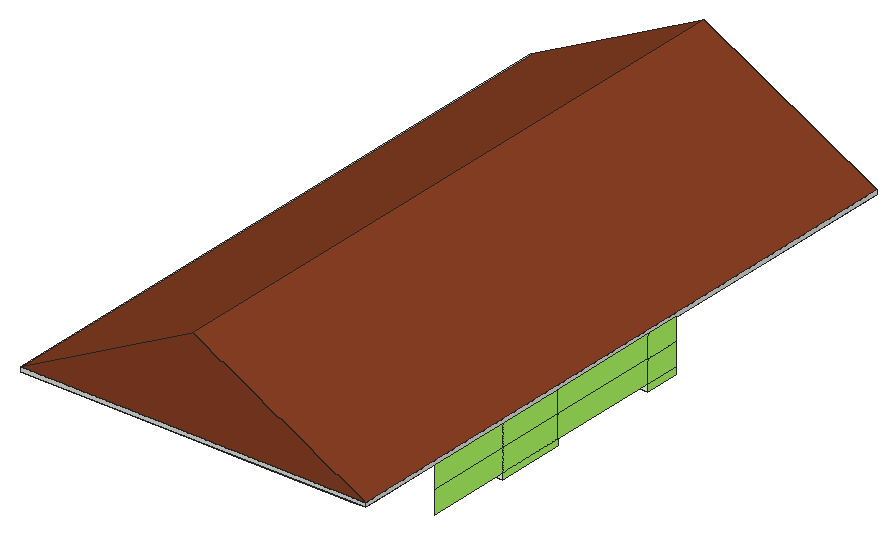
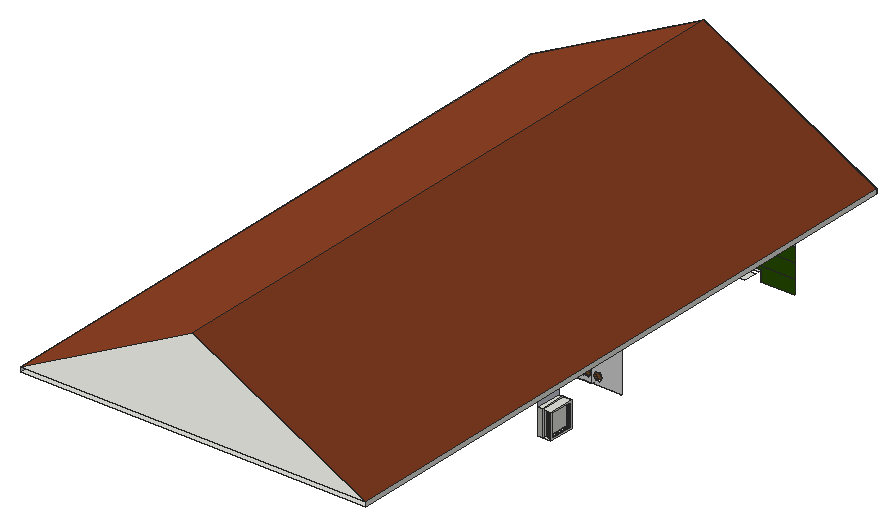
# SketchUp Ruby script. Lengths in inches.
U = 1.inch
M = Sketchup.active_model
def pt(a) = Geom::Point3d.new(a.map { |v| v * U })
def face(e, loops, mat)
  f = e.add_face(loops[0].map { |a| pt(a) })
  loops[1..].each { |l| e.add_face(l.map { |a| pt(a) }).erase! }
  f.material = f.back_material = mat if mat
  f
end
# faces: each face lists its corners as indices into pts; further lists are holes
def faces(e, pts, list, mat = nil) = list.each { |f| face(e, (f[0].is_a?(Array) ? f : [f]).map { |l| l.map { |i| pts[i] } }, mat) }
# xy, xz, yz: faces in a plane at the given z, y or x. An outline is a flat list of corners, or four numbers for a rectangle; further outlines are holes
def ring(l) = l.size == 4 ? [[l[0], l[1]], [l[2], l[1]], [l[2], l[3]], [l[0], l[3]]] : l.each_slice(2).to_a
def flat(e, list, mat, &to3) = list.each { |f| face(e, (f[0].is_a?(Array) ? f : [f]).map { |l| ring(l).map { |u, v| to3.(u, v) } }, mat) }
def xy(e, z, list, mat = nil) = flat(e, list, mat) { |x, y| [x, y, z] }
def xz(e, y, list, mat = nil) = flat(e, list, mat) { |x, z| [x, y, z] }
def yz(e, x, list, mat = nil) = flat(e, list, mat) { |y, z| [x, y, z] }
def lines(e, pts, list) = list.each { |a, b| e.add_line(pt(pts[a]), pt(pts[b])) }
# prism: a flat outline (further loops are holes) pulled along v
def prism(e, loops, v, mat = nil)
  f = face(e, loops, mat); d = Geom::Vector3d.new(v.map { |x| x * U })
  f.pushpull(f.normal.samedirection?(d) ? d.length : -d.length)
end
def box(e, o, s, mat = nil) = prism(e, [[o, [o[0] + s[0], o[1], o[2]], [o[0] + s[0], o[1] + s[1], o[2]], [o[0], o[1] + s[1], o[2]]]], [0, 0, s[2]], mat)
def at(x, y, z, deg = 0) = Geom::Transformation.translation(pt([x, y, z])) * Geom::Transformation.rotation(ORIGIN, Z_AXIS, deg.degrees)
def axes(o, x, y, z) = Geom::Transformation.new([*x, 0, *y, 0, *z, 0, *pt(o).to_a, 1])
def part(name) = M.definitions.add(name)
# library, detail: a bought-in or finely detailed component or shape, given as its bounding box
def library(name, o, s) = part(name).tap { |d| box(d.entities, o, s) }
def detail(e, o, s) = box(e.add_group.entities, o, s)
def put(e, d, t, mat = nil) = e.add_instance(d, t).tap { |i| i.material = mat if mat }
def group(e, t, mat = nil) = e.add_group.tap { |g| g.transformation = t; g.material = mat if mat }.entities
root = M.entities
M.materials.add("[Color F01]").color = [47, 96, 0]
M.materials.add("[Color F03]").color = [178, 255, 101]
M.materials.add("[Color K01]").color = [255, 204, 255]
M.materials.add("[Color M00]").color = [255, 255, 255]
M.materials.add("[Color M09]").color = [0, 0, 0]
M.materials.add("[Marble Carrara Floor Tile]").color = [204, 208, 219]
M.materials.add("[Roofing Tile Spanish]").color = [138, 64, 36]
M.materials.add("[Wood Cherry Original]").color = [152, 86, 42]
M.materials.add("[Wood Floor Parquet]").color = [145, 89, 39]
c1 = part("Copyright 2018, ")
xy(c1.entities,0.05,[[[19.06,0,19.06,9.82,21.3125,9.82,22.13,9.76,22.85,9.6,23.48,9.33,24,8.95,24.43,8.48,24.73,7.92,24.91,7.28,24.97,6.54,24.91,5.85,24.74,5.21,24.46,4.64,24.0625,4.14,23.58,3.73,23.03,3.4375,22.42,3.26,21.75,3.2,21.1,3.27,20.375,3.48,20.375,0],[21.62,4.3125,22.05,4.35,22.4375,4.47,22.79,4.66,23.09,4.94,23.34,5.28,23.52,5.66,23.63,6.09,23.67,6.56,23.6,7.16,23.4,7.68,23.08,8.1,22.66,8.39,22.08,8.56,21.28,8.61,20.375,8.61,20.375,4.61,20.98,4.39]],[25.77,0,27.98,4.71,25.47,9.82,26.9375,9.82,28.69,6.14,30.375,9.82,31.82,9.82,27.21,0],[[43.77,0,43.11,0.03,42.52,0.14,41.99,0.3125,41.54,0.55,41.18,0.86,40.92,1.2,40.77,1.6,40.71,2.04,40.82,2.64,41.12,3.13,41.63,3.5,42.35,3.75,41.86,4.16,41.74,4.37,41.7,4.57,41.77,4.87,41.98,5.14,42.3,5.36,42.73,5.51,42.1,5.88,41.65,6.34,41.38,6.91,41.29,7.57,41.34,8.0625,41.48,8.5,41.72,8.88,42.05,9.21,42.47,9.48,42.95,9.67,43.5,9.78,44.13,9.82,46.81,9.82,46.81,8.8125,45.49,8.8125,46.02,8.11,46.13,7.77,46.17,7.38,46.1,6.875,45.88,6.38,45.55,5.94,45.13,5.625,44.53,5.39,43.64,5.21,43.09,5.03,42.96,4.89,42.91,4.71,42.98,4.5,43.18,4.34,44.17,4.04,45.71,3.625,46.33,3.2,46.67,2.67,46.79,2.03,46.74,1.59,46.59,1.2,46.33,0.85,45.97,0.55,45.52,0.31,45.01,0.14,44.42,0.03],[43.74,1.02,44.5,1.09,45.0625,1.28,45.42,1.58,45.53,1.99,45.5,2.2,45.39,2.4,44.94,2.72,44.26,2.9375,43.41,3.01,42.82,2.94,42.34,2.73,42.03,2.42,41.93,2.03,42.04,1.59,42.38,1.28,42.95,1.09],[43.72,6.34,44.22,6.42,44.63,6.67,44.91,7.05,45,7.51,44.9,7.98,44.63,8.36,44.22,8.61,43.71,8.7,43.23,8.61,42.82,8.35,42.54,7.96,42.45,7.5,42.54,7.04,42.8125,6.67,43.22,6.42]],[180.16,0,182.36,4.71,179.85,9.82,181.32,9.82,183.07,6.14,184.75,9.82,186.2,9.82,181.59,0],[[219.8,0,219.13,0.03,218.54,0.14,218.02,0.3125,217.57,0.55,217.21,0.86,216.95,1.2,216.79,1.6,216.74,2.04,216.84,2.64,217.15,3.13,217.66,3.5,218.375,3.75,217.89,4.16,217.77,4.37,217.72,4.57,217.79,4.87,218,5.14,218.33,5.36,218.76,5.51,218.13,5.88,217.68,6.34,217.41,6.91,217.32,7.57,217.37,8.0625,217.51,8.5,217.75,8.88,218.08,9.21,218.5,9.48,218.98,9.67,219.53,9.78,220.16,9.82,222.83,9.82,222.83,8.8125,221.52,8.8125,222.05,8.11,222.16,7.77,222.2,7.38,222.125,6.875,221.91,6.38,221.58,5.94,221.16,5.625,220.5625,5.39,219.67,5.21,219.12,5.03,218.99,4.89,218.94,4.71,219.01,4.5,219.21,4.34,220.2,4.04,221.73,3.625,222.35,3.2,222.7,2.67,222.82,2.03,222.77,1.59,222.61,1.2,222.36,0.85,222,0.55,221.55,0.31,221.03,0.14,220.45,0.03],[219.77,1.02,220.53,1.09,221.09,1.28,221.44,1.58,221.5625,1.99,221.52,2.2,221.41,2.4,220.97,2.72,220.29,2.9375,219.43,3.01,218.84,2.94,218.37,2.73,218.0625,2.42,217.96,2.03,218.07,1.59,218.41,1.28,218.98,1.09],[219.75,6.34,220.25,6.42,220.66,6.67,220.93,7.05,221.02,7.51,220.93,7.98,220.66,8.36,220.24,8.61,219.74,8.7,219.25,8.61,218.85,8.35,218.57,7.96,218.48,7.5,218.57,7.04,218.84,6.67,219.25,6.42]],
  [92.62,1.6,92.62,1.87,92.89,2.17,93.07,2.48,93.22,3.3125,92.89,3.45,92.65,3.66,92.51,3.92,92.47,4.24,92.53,4.6,92.72,4.9,93.01,5.11,93.34,5.18,93.73,5.08,94.04,4.8,94.25,4.36,94.32,3.82,94.2,3.09,93.87,2.45,93.33,1.9375],[6.01,3.2,5.21,3.24,4.48,3.37,3.81,3.58,3.2,3.87,2.66,4.23,2.17,4.66,1.74,5.14,1.38,5.7,1.08,6.29,0.875,6.91,0.75,7.55,0.71,8.22,0.8,9.25,1.09,10.2,1.57,11.07,2.24,11.84,3.06,12.49,3.96,12.95,4.95,13.22,6.04,13.3125,6.83,13.26,7.68,13.11,8.5625,12.86,9.49,12.5,9.49,10.98,8.63,11.42,7.78,11.72,6.9375,11.91,6.11,11.97,5.29,11.9,4.55,11.7,3.89,11.37,3.29,10.9,2.8,10.33,2.45,9.7,2.24,8.99,2.17,8.22,2.24,7.44,2.45,6.74,2.79,6.11,3.27,5.55,3.86,5.09,4.53,4.76,5.27,4.57,6.09,4.5,6.98,4.57,7.87,4.78,8.74,5.12,9.6,5.6,9.6,4.05,8.79,3.68,7.92,3.41,6.99,3.25],[[14.21,3.2,13.51,3.26,12.87,3.4375,12.29,3.73,11.77,4.14,11.34,4.65,11.03,5.21,10.85,5.82,10.78,6.5,10.85,7.1875,11.03,7.81,11.34,8.375,11.78,8.88,12.31,9.3,12.9,9.59,13.55,9.77,14.27,9.83,14.98,9.77,15.63,9.59,16.21,9.29,16.73,8.87,17.16,8.36,17.47,7.79,17.66,7.16,17.72,6.47,17.66,5.79,17.47,5.18,17.16,4.625,16.72,4.13,16.19,3.72,15.6,3.43,14.9375,3.26],[14.25,4.4,14.71,4.44,15.12,4.55,15.48,4.74,15.81,5,16.07,5.32,16.26,5.68,16.37,6.08,16.41,6.53,16.37,6.97,16.25,7.375,16.06,7.74,15.78,8.0625,15.45,8.33,15.07,8.52,14.65,8.63,14.2,8.67,13.76,8.63,13.36,8.52,13,8.33,12.68,8.0625,12.42,7.74,12.23,7.37,12.12,6.97,12.08,6.52,12.12,6.07,12.24,5.67,12.43,5.31,12.69,4.99,13.02,4.73,13.39,4.55,13.8,4.44]],[57.3125,3.2,56.51,3.33,55.84,3.72,55.54,4.07,55.34,4.58,55.26,5.77,55.26,8.66,54.13,8.66,54.13,8.78,56.54,11.16,56.54,9.82,58.6,9.82,58.6,8.66,56.54,8.66,56.54,5.48,56.6,4.99,56.78,4.64,57.06,4.43,57.47,4.36,58.18,4.48,58.93,4.82,58.93,3.62,58.16,3.31],[[88.3125,3.2,87.67,3.25,87.08,3.41,86.54,3.66,86.06,4.02,85.66,4.45,85.37,4.93,85.2,5.46,85.14,6.04,85.23,6.75,85.49,7.37,85.93,7.91,86.54,8.36,86,8.86,85.64,9.37,85.4375,9.91,85.37,10.54,85.43,11.1,85.59,11.61,85.86,12.08,86.24,12.51,86.7,12.86,87.21,13.11,87.76,13.26,88.37,13.3125,88.96,13.26,89.51,13.11,90.01,12.86,90.46,12.51,90.83,12.09,91.09,11.62,91.25,11.1,91.31,10.54,91.23,9.91,91,9.33,90.62,8.82,90.08,8.36,90.68,7.91,91.11,7.38,91.36,6.75,91.45,6.02,91.39,5.4375,91.23,4.91,90.95,4.43,90.56,4,90.08,3.65,89.55,3.4,88.96,3.25],[88.33,4.54,89,4.64,89.54,4.94,89.9,5.39,90.02,5.96,90.02,6.11,89.9,6.72,89.54,7.21,88.98,7.53,88.28,7.64,87.6,7.53,87.05,7.21,86.69,6.71,86.57,6.09,86.69,5.47,87.06,4.98,87.62,4.65],[88.35,9.02,88.95,9.125,89.45,9.45,89.79,9.93,89.9,10.49,89.79,11.08,89.46,11.55,88.96,11.87,88.34,11.97,87.72,11.87,87.22,11.5625,86.89,11.09,86.78,10.51,86.89,9.9375,87.24,9.46,87.75,9.13]],
  [[113.29,3.2,112.92,3.24,112.64,3.36,112.43,3.57,112.32,3.85,111.9,3.57,111.47,3.375,111.03,3.26,110.57,3.22,109.95,3.33,109.44,3.66,109.1,4.17,108.99,4.79,109.1,5.375,109.43,5.89,109.97,6.32,110.6875,6.66,112.33,7.22,112.33,7.57,112.26,8.08,112.04,8.45,111.67,8.67,111.16,8.74,110.64,8.67,110.12,8.47,109.61,8.13,109.11,7.65,109.11,9.06,109.53,9.45,110.02,9.72,110.6,9.89,111.27,9.94,111.77,9.91,112.21,9.81,112.61,9.63,112.95,9.39,113.34,8.92,113.55,8.34,113.6,7.22,113.6,4.46,113.65,4.21,113.82,4.13,114.12,4.21,114.55,4.47,114.55,3.6875,113.85,3.3],[111.19,4.1,111.79,4.22,112.33,4.6,112.33,6.53,111.47,6.2,110.91,5.9375,110.54,5.67,110.34,5.375,110.27,5.01,110.33,4.64,110.53,4.35,110.82,4.16]],[121.02,3.2,120.43,3.28,119.88,3.51,119.43,3.87,119.1,4.34,118.9,5.04,118.83,6.09,118.83,9.82,120.12,9.82,120.12,6.11,120.19,5.24,120.41,4.68,120.82,4.38,121.44,4.28,121.88,4.33,122.29,4.5,122.66,4.78,123,5.17,123,9.82,124.29,9.82,124.29,3.3125,123,3.3125,123,4.15,122.5625,3.75,122.07,3.45,121.54,3.26],[[156.36,3.2,155.99,3.24,155.7,3.36,155.5,3.57,155.39,3.85,154.97,3.57,154.54,3.375,154.1,3.26,153.64,3.22,153.02,3.33,152.51,3.66,152.17,4.17,152.06,4.79,152.17,5.375,152.5,5.89,153.03,6.32,153.75,6.66,155.4,7.22,155.4,7.57,155.33,8.08,155.11,8.45,154.74,8.67,154.23,8.74,153.7,8.67,153.1875,8.47,152.68,8.13,152.18,7.65,152.18,9.06,152.59,9.45,153.09,9.72,153.67,9.89,154.33,9.94,154.83,9.91,155.28,9.81,155.68,9.63,156.02,9.39,156.4,8.92,156.62,8.34,156.66,7.22,156.66,4.46,156.72,4.21,156.89,4.13,157.1875,4.21,157.62,4.47,157.62,3.6875,156.92,3.3],[154.26,4.1,154.85,4.22,155.4,4.6,155.4,6.53,154.54,6.2,153.98,5.9375,153.61,5.67,153.4,5.375,153.34,5.01,153.4,4.64,153.59,4.35,153.89,4.16]],[161.74,3.2,161.01,3.26,160.37,3.43,159.8,3.71,159.3,4.11,158.91,4.6,158.62,5.16,158.45,5.81,158.4,6.53,158.45,7.26,158.62,7.92,158.89,8.5,159.28,9,159.76,9.41,160.3,9.71,160.92,9.88,161.6,9.94,162.51,9.85,163.49,9.49,163.49,8.12,162.55,8.59,161.68,8.74,161.27,8.7,160.89,8.59,160.55,8.4,160.25,8.13,160.01,7.8,159.84,7.4375,159.73,7.02,159.7,6.57,159.73,6.1,159.85,5.68,160.04,5.31,160.3,4.99,160.63,4.73,161.01,4.55,161.44,4.4375,161.93,4.4,162.73,4.51,163.63,4.83,163.63,3.5625,162.67,3.29],[[178.37,3.2,178,3.24,177.71,3.36,177.51,3.57,177.39,3.85,176.98,3.57,176.55,3.375,176.1,3.26,175.65,3.22,175.02,3.33,174.52,3.66,174.18,4.17,174.0625,4.79,174.17,5.375,174.51,5.89,175.04,6.32,175.76,6.66,177.41,7.22,177.41,7.57,177.33,8.08,177.11,8.45,176.75,8.67,176.23,8.74,175.71,8.67,175.19,8.47,174.6875,8.13,174.18,7.65,174.18,9.06,174.6,9.45,175.1,9.72,175.68,9.89,176.34,9.94,176.84,9.91,177.29,9.81,177.68,9.63,178.03,9.39,178.41,8.92,178.625,8.34,178.67,7.22,178.67,4.46,178.73,4.21,178.9,4.13,179.2,4.21,179.625,4.47,179.625,3.6875,178.92,3.3],[176.27,4.1,176.86,4.22,177.41,4.6,177.41,6.53,176.54,6.2,175.98,5.9375,175.61,5.67,175.41,5.375,175.34,5.01,175.41,4.64,175.6,4.35,175.9,4.16]],
  [210.76,3.2,209.73,3.33,208.59,3.78,208.59,5.17,209.71,4.55,210.23,4.37,210.66,4.3125,211.04,4.36,211.36,4.51,211.57,4.73,211.65,4.98,211.6,5.24,211.46,5.45,210.65,5.99,209.62,6.64,209.02,7.18,208.73,7.69,208.64,8.25,208.67,8.6,208.78,8.93,208.96,9.22,209.22,9.47,209.89,9.83,210.72,9.94,211.6875,9.81,212.68,9.41,212.68,8.13,211.64,8.65,210.81,8.83,210.47,8.79,210.2,8.67,210.03,8.48,209.97,8.25,210.02,8.03,210.18,7.82,210.91,7.32,211.37,7.06,212.08,6.59,212.59,6.09,212.89,5.57,213,5.02,212.96,4.64,212.84,4.3,212.64,3.99,212.37,3.71,212.04,3.49,211.66,3.33],[[73.82,3.22,73.14,3.3,72.53,3.56,71.99,3.99,71.52,4.59,71.14,5.34,70.87,6.2,70.7,7.17,70.65,8.25,70.71,9.32,70.875,10.29,71.16,11.15,71.55,11.9,72.03,12.52,72.58,12.96,73.2,13.23,73.88,13.3125,74.53,13.23,75.12,12.96,75.65,12.51,76.125,11.89,76.51,11.13,76.79,10.27,76.96,9.32,77.01,8.28,76.96,7.2,76.79,6.24,76.51,5.38,76.125,4.62,75.65,4.01,75.11,3.57,74.5,3.3],[73.81,4.52,74.2,4.58,74.54,4.77,74.84,5.08,75.1,5.51,75.31,6.06,75.46,6.6875,75.58,8.22,75.46,9.76,75.32,10.4,75.12,10.95,74.87,11.4,74.59,11.72,74.26,11.91,73.89,11.97,73.82,11.97,73.4375,11.91,73.09,11.72,72.79,11.41,72.53,10.97,72.32,10.43,72.18,9.79,72.06,8.26,72.17,6.7,72.32,6.06,72.52,5.51,72.78,5.08,73.08,4.77,73.42,4.58]],[[204.86,3.22,203.89,3.33,203.125,3.66,202.53,4.18,202.06,4.86,201.76,5.67,201.66,6.6,201.71,7.31,201.87,7.95,202.13,8.51,202.5,9.01,202.95,9.42,203.47,9.71,204.05,9.89,204.6875,9.94,205.3,9.89,205.85,9.72,206.33,9.43,206.75,9.04,207.09,8.55,207.33,7.98,207.47,7.34,207.52,6.61,207.52,6.45,202.95,6.45,203.13,5.61,203.32,5.27,203.57,4.97,203.88,4.73,204.23,4.55,205.06,4.42,205.68,4.47,206.28,4.61,206.86,4.86,207.41,5.21,207.41,3.95,206.82,3.61,206.23,3.39,205.6,3.26],[202.98,7.22,206.25,7.22,206.11,7.9,205.79,8.41,205.31,8.72,204.6875,8.83,204.06,8.72,203.55,8.41,203.1875,7.9]],[32.81,3.3125,32.81,9.82,34.1,9.82,34.1,8.33,34.17,8.4375,34.64,9.1,35.1,9.57,35.57,9.85,36.04,9.94,36.4,9.9,36.78,9.76,37.55,9.21,36.875,8.08,36.23,8.55,35.63,8.71,35.33,8.68,35.05,8.57,34.55,8.12,34.21,7.47,34.1,6.71,34.1,3.3125],[38.48,3.3125,39.77,9.82],
  [47.77,3.3125,47.77,13.1875,49.06,13.1875,49.06,8.96,49.49,9.39,49.96,9.7,50.49,9.88,51.06,9.94,51.68,9.86,52.23,9.62,52.68,9.23,52.99,8.72,53.18,8.01,53.24,7.02,53.24,3.3125,51.96,3.3125,51.96,7.34,51.87,7.98,51.61,8.48,51.2,8.81,50.6875,8.92,50.27,8.86,49.89,8.7,49.49,8.41,49.06,7.97,49.06,3.3125],[63.46,3.3125,63.46,3.41,64.06,4.11,66.27,7.04,66.95,8.09,67.35,8.86,67.53,9.47,67.6,10.07,67.48,10.82,67.125,11.41,66.57,11.79,65.87,11.92,65.28,11.83,64.7,11.57,64.15,11.14,63.66,10.58,63.66,12.375,64.24,12.79,64.83,13.08,65.43,13.26,66.04,13.3125,66.65,13.26,67.21,13.1,67.72,12.83,68.17,12.45,68.53,11.99,68.79,11.47,68.95,10.9,69,10.26,68.95,9.65,68.8,8.99,68.51,8.27,68.06,7.4375,67.34,6.4,66.26,5.04,65.95,4.68,69.71,4.68,69.71,3.3125],[80.37,3.3125,81.78,13.1875],[100.21,3.3125,100.21,13.1875,101.625,13.1875,101.625,8.67,105.78,13.1875,107.55,13.1875,103.27,8.5,108.6,3.3125,106.67,3.3125,101.625,8.19,101.625,3.3125],[115.72,3.3125,117,13.1875],
  [126.04,3.3125,126.04,9.82,127.33,9.82,127.33,8.96,127.82,9.39,128.3,9.7,128.78,9.88,129.25,9.94,129.83,9.87,130.35,9.65,130.79,9.28,131.17,8.77,131.6875,9.29,132.22,9.66,132.77,9.88,133.32,9.96,133.77,9.91,134.18,9.78,134.55,9.57,134.88,9.27,135.15,8.875,135.34,8.39,135.45,7.82,135.49,7.15,135.49,3.3125,134.2,3.3125,134.2,7.17,134.12,7.88,133.87,8.41,133.47,8.73,132.92,8.84,132.53,8.79,132.15,8.64,131.78,8.39,131.43,8.04,131.43,3.3125,130.13,3.3125,130.13,6.93,130.0625,7.85,129.84,8.44,129.67,8.63,129.45,8.76,128.83,8.87,128.45,8.82,128.1,8.6875,127.74,8.43,127.33,8.04,127.33,3.3125],[141.43,3.3125,141.43,13.1875,142.77,13.1875,146.05,9.13,149.31,13.1875,150.63,13.1875,150.63,3.3125,149.21,3.3125,149.21,11,146.17,7.18,145.91,7.18,142.84,11,142.84,3.3125],[165.29,3.3125,165.29,13.1875,166.7,13.1875,166.7,8.67,170.86,13.1875,172.62,13.1875,168.34,8.5,173.67,3.3125,171.75,3.3125,166.7,8.19,166.7,3.3125],[214.51,3.3125,215.8,9.82],[223.8,3.3125,223.8,9.82,225.12,9.82,225.12,8.99,225.5625,9.41,226.04,9.7,226.54,9.88,227.07,9.94,227.66,9.86,228.2,9.63,228.67,9.26,229,8.77,229.2,8.06,229.27,7.03,229.27,3.3125,227.99,3.3125,227.99,7.02,227.91,7.87,227.68,8.44,227.28,8.76,226.66,8.87,226.23,8.8125,225.82,8.64,225.45,8.36,225.12,7.96,225.12,3.3125],
  [[191.3125,3.33,191.3125,13.1875,194.64,13.1875,195.6,13.15,196.45,13.04,197.19,12.85,197.83,12.58,198.39,12.25,198.88,11.84,199.32,11.36,199.7,10.81,200,10.21,200.22,9.58,200.35,8.93,200.39,8.25,200.29,7.28,200.01,6.35,199.54,5.5,198.92,4.76,198.14,4.14,197.24,3.7,196.22,3.4,194.4375,3.33],[192.73,4.59,194.54,4.59,195.48,4.62,196.18,4.73,197.16,5.1,197.88,5.65,198.34,6.21,198.66,6.85,198.86,7.55,198.93,8.33,198.86,9.08,198.66,9.77,198.32,10.38,197.85,10.92,197.43,11.26,196.94,11.53,195.97,11.85,194.49,11.93,192.73,11.93]],[39.12,11.03,38.84,11.09,38.59,11.26,38.42,11.51,38.37,11.8,38.42,12.08,38.59,12.32,38.84,12.49,39.12,12.55,39.41,12.5,39.66,12.33,39.83,12.09,39.89,11.8,39.83,11.51,39.66,11.26,39.41,11.09],[215.14,11.03,214.87,11.09,214.62,11.26,214.45,11.51,214.4,11.8,214.45,12.08,214.62,12.32,214.87,12.49,215.14,12.55,215.44,12.5,215.6875,12.33,215.86,12.09,215.92,11.8,215.86,11.51,215.6875,11.26,215.44,11.09]])
xy(root,122.43,[[36.01,60,84.01,69],[151.25,60,151.5,69],[151.5,60,187.5,69],[99,234,129,238.5],[231,245.63,240,269.63],
  [93,250.5,97.5,286.5]])
xy(root,123.43,[[231,118.97,240,166.97]])
xy(root,124.43,[[34.01,58,86.01,60]])
xy(root,125.32,[[24.2,208.375,27.2,210]],"[Color M00]")
xy(root,125.4375,[[67.38,208.5,70.38,210]],"[Color K01]")
xy(root,125.4375,[[32.14,208.5,35.14,210]],"[Color M00]")
xy(root,125.49,[[73.875,208.5,76.82,210]],"[Color K01]")
xy(root,126.43,[[32.01,58,88.01,60]])
xy(root,128.44,[[0,264.68,6,282.68]])
xy(root,129.3125,[[0,265.55,1.25,281.8125],[4.75,265.55,6,281.8125]])
xy(root,129.57,[[1.25,265.81,2.5,281.56],[2.5,265.81,3.5,281.56],[3.5,265.81,4.75,281.56]])
xy(root,129.78,[[2.5,266.02,2.6,281.34],[2.6,266.02,3.4,281.34],[3.4,266.02,3.5,281.34]])
xy(root,130.52,[[24.2,208.375,27.2,210]],"[Wood Floor Parquet]")
xy(root,130.59,[[73.875,208.5,76.82,210]],"[Wood Floor Parquet]")
xy(root,130.63,[[32.14,208.5,35.14,210],[67.38,208.5,70.38,210]],"[Wood Floor Parquet]")
xy(root,145.09,[[2.5,266.02,2.6,281.34],[2.6,266.02,3.4,281.34],[3.4,266.02,3.5,281.34]])
xy(root,145.31,[[1.25,265.81,2.5,281.56],[2.5,265.81,3.5,281.56],[3.5,265.81,4.75,281.56]])
xy(root,145.5625,[[0,265.55,1.25,281.8125],[4.75,265.55,6,281.8125]])
xy(root,146.43,[[0,264.68,6,282.68],[6,264.68,9,282.68]])
xy(root,158.43,[[0,0,0,57,9,57,9,60,133.5,60,133.5,0],[133.5,0,141.5,8],[141.5,0,232,60],[232,0,240,8],[133.5,8,141.5,52],
  [232,8,240,52],[133.5,52,141.5,60],[232,52,240,60],[[0,57,9,57,9,60,133.5,60,133.5,234,140.7,234,140.7,238.5,97.5,238.5,97.5,298.5,140.7,298.5,140.7,303,133.5,303,133.5,435,231,435,231,303,164.7,303,164.7,298.5,231,298.5,231,69,133.5,69,133.5,60,240,60,240,444,0,444],[9,69,129,234],[9,303,129,435],[9,238.5,93,298.5]]])
xy(root,158.43,[[9,210,93,234]],"[Wood Cherry Original]")
xy(root,161.43,[[0,0,240,444]])
xz(root,0,[[0,158.43,240,161.43]])
xz(root,0,[[0,161.43,240,161.43,120,224.68]],"[Roofing Tile Spanish]")
xz(root,60,[[9,148.43,133.5,158.43]])
xz(root,60,[[9,118.43,32.01,118.43,32.01,126.43,88.01,126.43,88.01,118.43,133.5,118.43,133.5,128.43,9,128.43],[9,128.43,133.5,138.43],[9,138.43,133.5,148.43]],"[Color F01]")
xz(root,208.375,[[24.2,125.32,27.2,125.32,28.7,127.92,27.2,130.52,24.2,130.52,22.7,127.92]],"[Wood Floor Parquet]")
xz(root,208.5,[[32.14,125.4375,35.14,125.4375,36.64,128.04,35.14,130.63,32.14,130.63,30.64,128.04],[67.38,125.4375,70.38,125.4375,71.88,128.04,70.38,130.63,67.38,130.63,65.88,128.04],[73.875,125.49,76.82,125.49,78.29,128.04,76.82,130.59,73.875,130.59,72.4,128.04]],"[Wood Floor Parquet]")
xz(root,210,[[[51.3,122.43,72,158.43],[67.38,125.4375,65.88,128.04,67.38,130.63,70.38,130.63,71.88,128.04,70.38,125.4375]],[[72.3,122.43,93,158.43],[73.875,125.49,72.4,128.04,73.875,130.59,76.82,130.59,78.29,128.04,76.82,125.49]]],"[Color K01]")
xz(root,210,[[[9,122.43,30,158.43],[24.2,125.32,22.7,127.92,24.2,130.52,27.2,130.52,28.7,127.92,27.2,125.32]],[[30.3,122.43,51,158.43],[32.14,125.4375,30.64,128.04,32.14,130.63,35.14,130.63,36.64,128.04,35.14,125.4375]]],"[Color M00]")
xz(root,210,[[9,122.13,30,122.43],[30.3,122.13,51,122.43],[51.3,122.13,72,122.43],[72.3,122.13,93,122.43]],"[Color M09]")
xz(root,264.68,[[9,128.43,6,128.44,6,146.43,9,146.43],[0,128.44,6,146.43]])
xz(root,265.55,[[0,129.3125,1.25,145.5625],[4.75,129.3125,6,145.5625]])
xz(root,265.81,[[1.25,129.57,2.5,145.31],[2.5,129.57,3.5,145.31],[3.5,129.57,4.75,145.31]])
xz(root,266.02,[[2.5,129.78,2.6,145.09],[2.6,129.78,3.4,145.09],[3.4,129.78,3.5,145.09]])
xz(root,281.34,[[2.5,129.78,2.6,145.09],[2.6,129.78,3.4,145.09],[3.4,129.78,3.5,145.09]])
xz(root,281.56,[[1.25,129.57,2.5,145.31],[2.5,129.57,3.5,145.31],[3.5,129.57,4.75,145.31]])
xz(root,281.8125,[[0,129.3125,1.25,145.5625],[4.75,129.3125,6,145.5625]])
xz(root,282.68,[[9,128.43,9,146.43,6,146.43,6,128.44]])
yz(root,0,[[[264.68,128.44,282.68,146.43],[265.55,129.3125,281.8125,145.5625]],[0,158.43,444,161.43]])
yz(root,1.25,[[[265.55,129.3125,281.8125,145.5625],[265.81,129.57,281.56,145.31]]])
yz(root,2.5,[[[265.81,129.57,281.56,145.31],[266.02,129.78,281.34,145.09]]])
yz(root,2.6,[[266.02,129.78,281.34,145.09]])
yz(root,3.4,[[266.02,129.78,281.34,145.09]])
yz(root,3.5,[[[265.81,129.57,281.56,145.31],[266.02,129.78,281.34,145.09]]])
yz(root,4.75,[[[265.55,129.3125,281.8125,145.5625],[265.81,129.57,281.56,145.31]]])
yz(root,6,[[[264.68,128.44,282.68,146.43],[265.55,129.3125,281.8125,145.5625]]])
yz(root,9,[[264.68,146.43,282.68,158.43]],"[Marble Carrara Floor Tile]")
yz(root,32.01,[[58,118.43,60,126.43]])
yz(root,86.01,[[58,118.43,60,124.43]])
yz(root,88.01,[[58,118.43,60,126.43]])
yz(root,240,[[0,158.43,444,161.43]])
yz(root,240,[[245.63,122.43,269.63,127.68],[118.97,123.43,166.97,127.68],[60,127.68,118.97,143.06],[118.97,127.68,166.97,143.06],[166.97,127.68,245.63,143.06],
  [245.63,127.68,269.63,143.06],[60,143.06,118.97,158.43],[118.97,143.06,166.97,158.43],[166.97,143.06,245.63,158.43],[245.63,143.06,269.63,158.43]],"[Color F03]")
p = [[22.7,210,127.92],[24.2,210,125.32],[24.2,208.375,125.32],[22.7,208.375,127.92],[27.2,210,125.32],[28.7,210,127.92],
  [28.7,208.375,127.92],[27.2,208.375,125.32],[30.64,210,128.04],[32.14,210,125.4375],[32.14,208.5,125.4375],[30.64,208.5,128.04],
  [35.14,210,125.4375],[36.64,210,128.04],[36.64,208.5,128.04],[35.14,208.5,125.4375],[65.88,210,128.04],[67.38,210,125.4375],
  [67.38,208.5,125.4375],[65.88,208.5,128.04],[70.38,210,125.4375],[71.88,210,128.04],[71.88,208.5,128.04],[70.38,208.5,125.4375],
  [72.4,210,128.04],[73.875,210,125.49],[73.875,208.5,125.49],[72.4,208.5,128.04],[76.82,210,125.49],[78.29,210,128.04],
  [78.29,208.5,128.04],[76.82,208.5,125.49],[24.2,210,130.52],[24.2,208.375,130.52],[27.2,210,130.52],[27.2,208.375,130.52],
  [32.14,210,130.63],[32.14,208.5,130.63],[35.14,210,130.63],[35.14,208.5,130.63],[67.38,210,130.63],[67.38,208.5,130.63],
  [70.38,210,130.63],[70.38,208.5,130.63],[73.875,210,130.59],[73.875,208.5,130.59],[76.82,210,130.59],[76.82,208.5,130.59],
  [6,282.68,128.44],[9,282.68,128.43],[9,264.68,128.43],[6,264.68,128.44],[0,0,161.43],[120,0,224.68],
  [120,444,224.68],[0,444,161.43],[240,0,161.43],[240,444,161.43],[235.5,166.97,123.43],[235.5,166.97,158.43],
  [235.5,245.63,122.43],[235.5,245.63,158.43]]
faces(root,p,[[0,1,2,3],[8,9,10,11]],"[Color M00]")
faces(root,p,[[4,5,6,7],[12,13,14,15],[16,17,18,19],[20,21,22,23],[24,25,26,27],[28,29,30,31],[32,0,3,33],[5,34,35,6],
  [36,8,11,37],[13,38,39,14],[40,16,19,41],[21,42,43,22],[44,24,27,45],[29,46,47,30]],"[Wood Floor Parquet]")
faces(root,p,[[48,49,50,51]])
faces(root,p,[[52,53,54,55],[53,56,57,54]],"[Roofing Tile Spanish]")
lines(root,p,[[58,59],[60,61]])
put(root,c1,axes([2.05,279.96,145.83],[0,-0.05602,0],[0.1494,0,0],[0,0,0.37475]))
put(root,c1,axes([1.78,267.41,128.44],[0,0.05602,0],[0.1494,0,0],[0,0,-0.37475]))
